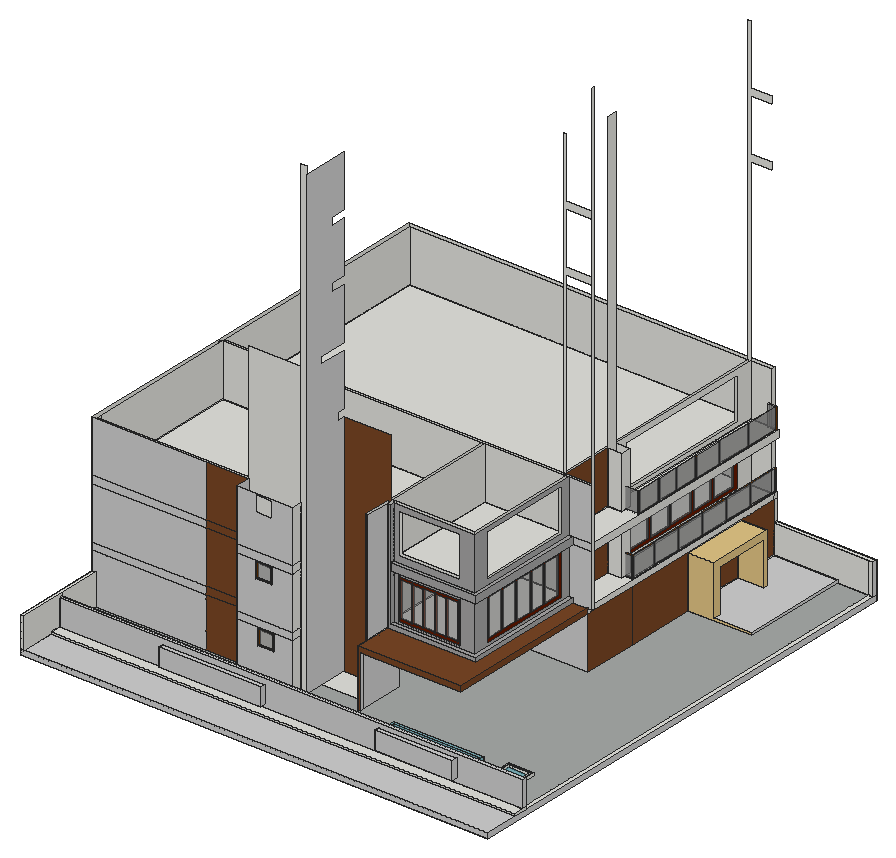
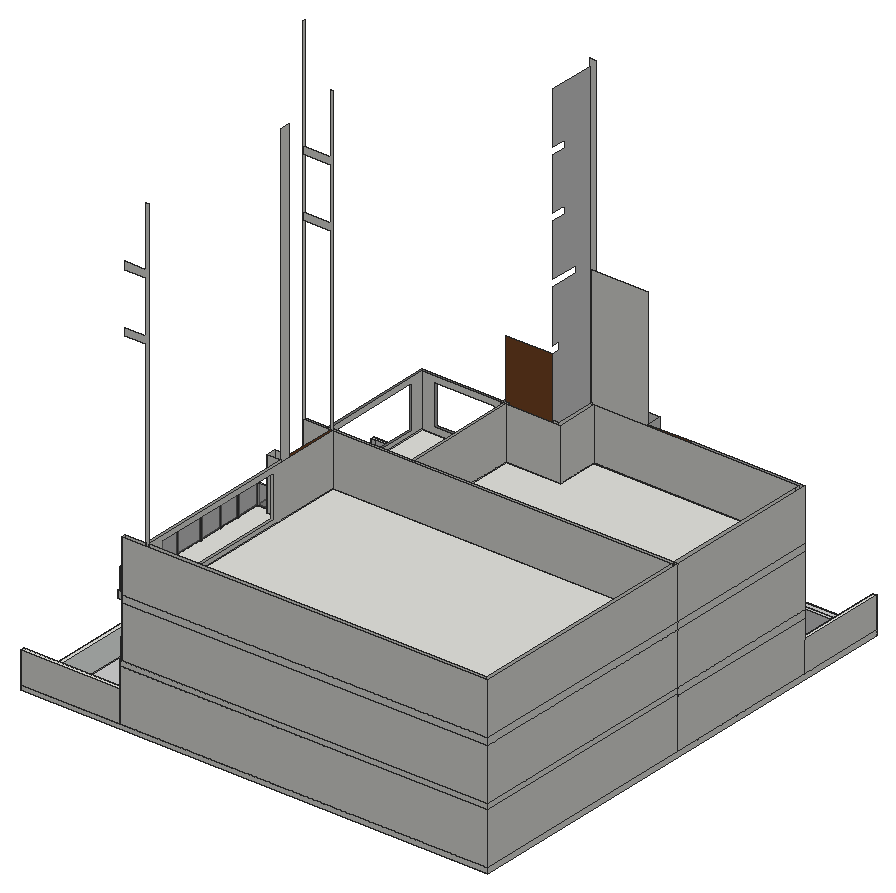
# SketchUp Ruby script. Lengths in inches.
U = 1.inch
M = Sketchup.active_model
def pt(a) = Geom::Point3d.new(a.map { |v| v * U })
def face(e, loops, mat)
  f = e.add_face(loops[0].map { |a| pt(a) })
  loops[1..].each { |l| e.add_face(l.map { |a| pt(a) }).erase! }
  f.material = f.back_material = mat if mat
  f
end
# faces: each face lists its corners as indices into pts; further lists are holes
def faces(e, pts, list, mat = nil) = list.each { |f| face(e, (f[0].is_a?(Array) ? f : [f]).map { |l| l.map { |i| pts[i] } }, mat) }
# xy, xz, yz: faces in a plane at the given z, y or x. An outline is a flat list of corners, or four numbers for a rectangle; further outlines are holes
def ring(l) = l.size == 4 ? [[l[0], l[1]], [l[2], l[1]], [l[2], l[3]], [l[0], l[3]]] : l.each_slice(2).to_a
def flat(e, list, mat, &to3) = list.each { |f| face(e, (f[0].is_a?(Array) ? f : [f]).map { |l| ring(l).map { |u, v| to3.(u, v) } }, mat) }
def xy(e, z, list, mat = nil) = flat(e, list, mat) { |x, y| [x, y, z] }
def xz(e, y, list, mat = nil) = flat(e, list, mat) { |x, z| [x, y, z] }
def yz(e, x, list, mat = nil) = flat(e, list, mat) { |y, z| [x, y, z] }
def lines(e, pts, list) = list.each { |a, b| e.add_line(pt(pts[a]), pt(pts[b])) }
# prism: a flat outline (further loops are holes) pulled along v
def prism(e, loops, v, mat = nil)
  f = face(e, loops, mat); d = Geom::Vector3d.new(v.map { |x| x * U })
  f.pushpull(f.normal.samedirection?(d) ? d.length : -d.length)
end
def box(e, o, s, mat = nil) = prism(e, [[o, [o[0] + s[0], o[1], o[2]], [o[0] + s[0], o[1] + s[1], o[2]], [o[0], o[1] + s[1], o[2]]]], [0, 0, s[2]], mat)
def at(x, y, z, deg = 0) = Geom::Transformation.translation(pt([x, y, z])) * Geom::Transformation.rotation(ORIGIN, Z_AXIS, deg.degrees)
def axes(o, x, y, z) = Geom::Transformation.new([*x, 0, *y, 0, *z, 0, *pt(o).to_a, 1])
def part(name) = M.definitions.add(name)
# library, detail: a bought-in or finely detailed component or shape, given as its bounding box
def library(name, o, s) = part(name).tap { |d| box(d.entities, o, s) }
def detail(e, o, s) = box(e.add_group.entities, o, s)
def put(e, d, t, mat = nil) = e.add_instance(d, t).tap { |i| i.material = mat if mat }
def group(e, t, mat = nil) = e.add_group.tap { |g| g.transformation = t; g.material = mat if mat }.entities
root = M.entities
M.materials.add("[Carrera Marble]").color = [207, 207, 207]
M.materials.add("[Color B08]").color = [102, 25, 0]
M.materials.add("[Color C08]").color = [102, 51, 0]
M.materials.add("[Concrete Form 4x8]").color = [167, 170, 168]
M.materials.add("[Stone Brushed Khaki]").color = [226, 197, 133]
M.materials.add("[Stone Vein Gray]").color = [166, 165, 165]
M.materials.add("[Translucent Glass Gray]").color = [128, 128, 128]
M.materials["[Translucent Glass Gray]"].alpha = 0.5
M.materials.add("[Water Pool Light]").color = [64, 149, 167]
M.materials["[Water Pool Light]"].alpha = 0.6
M.materials.add("[Wood Veneer 01]").color = [120, 70, 37]
c1 = part("Group\#1")
xy(c1.entities,0,[[0,0,21.625,260.4375]],"[Color C08]")
xy(c1.entities,20.42,[[0,20.42,21.625,240.02]],"[Color C08]")
xy(c1.entities,312.95,[[0,20.42,21.625,240.02]],"[Color C08]")
xy(c1.entities,333.375,[[0,0,21.625,260.4375]],"[Color C08]")
xz(c1.entities,0,[[0,0,21.625,333.375]],"[Color C08]")
xz(c1.entities,20.42,[[0,20.42,21.625,312.95]],"[Color C08]")
xz(c1.entities,240.02,[[0,20.42,21.625,312.95]],"[Color C08]")
xz(c1.entities,260.4375,[[0,0,21.625,333.375]],"[Color C08]")
yz(c1.entities,0,[[[0,0,260.4375,333.375],[20.42,20.42,240.02,312.95]]],"[Color C08]")
yz(c1.entities,21.625,[[[0,0,260.4375,333.375],[20.42,20.42,240.02,312.95]]],"[Color C08]")
yz(c1.entities,21.625,[[20.42,20.42,240.02,312.95]],"[Translucent Glass Gray]")
c2 = part("Group\#3")
xy(c2.entities,0,[[0,0,23.0625,440.625]],"[Color B08]")
xy(c2.entities,14.28,[[0,14.28,23.0625,92.65],[0,98.4,23.0625,173.71],[0,179.46,23.0625,261.65],[0,267.4,23.0625,340.59],[0,346.34,23.0625,426.35]],"[Color B08]")
xy(c2.entities,204.03,[[0,14.28,23.0625,92.65],[0,98.4,23.0625,173.71],[0,179.46,23.0625,261.65],[0,267.4,23.0625,340.59],[0,346.34,23.0625,426.35]],"[Color B08]")
xy(c2.entities,218.3125,[[0,0,23.0625,440.625]],"[Color B08]")
xz(c2.entities,0,[[0,0,23.0625,218.3125]],"[Color B08]")
xz(c2.entities,14.28,[[0,14.28,23.0625,204.03]],"[Color B08]")
xz(c2.entities,92.65,[[0,14.28,23.0625,204.03]],"[Color B08]")
xz(c2.entities,98.4,[[0,14.28,23.0625,204.03]],"[Color B08]")
xz(c2.entities,173.71,[[0,14.28,23.0625,204.03]],"[Color B08]")
xz(c2.entities,179.46,[[0,14.28,23.0625,204.03]],"[Color B08]")
xz(c2.entities,261.65,[[0,14.28,23.0625,204.03]],"[Color B08]")
xz(c2.entities,267.4,[[0,14.28,23.0625,204.03]],"[Color B08]")
xz(c2.entities,340.59,[[0,14.28,23.0625,204.03]],"[Color B08]")
xz(c2.entities,346.34,[[0,14.28,23.0625,204.03]],"[Color B08]")
xz(c2.entities,426.35,[[0,14.28,23.0625,204.03]],"[Color B08]")
xz(c2.entities,440.625,[[0,0,23.0625,218.3125]],"[Color B08]")
yz(c2.entities,0,[[[0,0,440.625,218.3125],[179.46,14.28,261.65,204.03],[346.34,14.28,426.35,204.03],[14.28,14.28,92.65,204.03],[98.4,14.28,173.71,204.03],[267.4,14.28,340.59,204.03]]],"[Color B08]")
yz(c2.entities,23.0625,[[[0,0,440.625,218.3125],[179.46,14.28,261.65,204.03],[346.34,14.28,426.35,204.03],[14.28,14.28,92.65,204.03],[98.4,14.28,173.71,204.03],[267.4,14.28,340.59,204.03]]],"[Color B08]")
yz(c2.entities,23.0625,[[14.28,14.28,92.65,204.03],[98.4,14.28,173.71,204.03],[179.46,14.28,261.65,204.03],[267.4,14.28,340.59,204.03],[346.34,14.28,426.35,204.03]],"[Translucent Glass Gray]")
xy(root,0,[[0,0,1080,1120.6875]])
xy(root,12,[[0,0,9,207.0625],[9,77.625,1080,109.6875],[[954.49,109.6875,1012.49,215.5625],[958.9,114.1,1008.08,211.15]],[1071,109.6875,1080,1111.6875],[362.25,171.6875,491.3125,207.0625],
  [491.3125,195.6875,506.0625,231.25],[[0,207.0625,0,573,9,573,9,322.75,491.3125,322.75,491.3125,207.0625],[9,213.0625,482.6875,316.75]],[613.75,207.0625,619.75,261.625],[9,213.0625,482.6875,316.75],[491.3125,231.25,506.0625,236.75],
  [491.3125,236.75,506.0625,301.1875],[506.0625,236.75,607.75,301.1875],[607.75,236.75,613.75,236.75,613.75,316.75,599,316.75,599,301.1875,607.75,301.1875],[613.75,261.625,619.75,316.75],[491.3125,301.1875,491.3125,322.75,613.75,322.75,613.75,316.75,599,316.75,599,301.1875],
  [[0,573,851.0625,1120.6875],[9,579,845.0625,1111.6875]],[9,579,845.0625,1111.6875],[851.0625,863.43,997.2,1111.6875],[851.0625,1111.6875,1080,1120.6875]])
xy(root,12,[[9,0,1080,77.625]],"[Carrera Marble]")
xy(root,12,[[[9,109.6875,954.49,109.6875,954.49,215.5625,1012.49,215.5625,1012.49,109.6875,1071,109.6875,1071,1111.6875,997.2,1111.6875,997.2,863.43,851.0625,863.43,851.0625,573,9,573,9,322.75,613.75,322.75,613.75,316.75,619.75,316.75,619.75,207.0625,613.75,207.0625,613.75,236.75,506.0625,236.75,506.0625,195.6875,491.3125,195.6875,491.3125,171.6875,362.25,171.6875,362.25,207.0625,9,207.0625],[733.15,114.31,932.85,161.57]]],"[Concrete Form 4x8]")
xy(root,12,[[958.9,114.1,1008.08,211.15]],"[Water Pool Light]")
xy(root,12.125,[[[728.53,109.6875,937.46,166.1875],[733.15,114.31,932.85,161.57]]])
xy(root,17,[[[954.49,109.6875,1012.49,215.5625],[958.9,114.1,1008.08,211.15]]])
xy(root,17.3125,[[9,77.625,1080,101.34],[9,101.34,1080,109.6875]])
xy(root,17.3125,[[911.25,863.43,997.2,863.43,997.2,1111.6875,851.0625,1111.6875,851.0625,1016.2,911.25,1016.2,911.25,1007.16,851.0625,1007.16,851.0625,881.2,911.25,881.2]],"[Carrera Marble]")
xy(root,23.48,[[248.24,89.97,482.8,101.34]],"[Carrera Marble]")
xy(root,25.83,[[745.92,89.41,925.92,101.34]],"[Carrera Marble]")
xy(root,44.9375,[[[728.53,109.6875,937.46,166.1875],[733.15,114.31,932.85,161.57]]],"[Water Pool Light]")
xy(root,64.42,[[248.24,89.97,482.8,101.34]],"[Carrera Marble]")
xy(root,67.2,[[745.92,89.41,925.92,101.34]],"[Carrera Marble]")
xy(root,76.6875,[[9,101.34,1080,109.6875]],"[Carrera Marble]")
xy(root,84,[[0,0,9,207.0625],[851.0625,1111.6875,1080,1120.6875]])
xy(root,88.1,[[410.19,171.6875,447.63,177.25]])
xy(root,116.5,[[851.0625,881.2,911.25,1007.16]])
xy(root,125.54,[[410.19,171.6875,447.63,177.25]])
xy(root,127,[[362.25,171.6875,491.3125,171.6875,491.3125,322.75,9,322.75,9,573,0,573,0,207.0625,362.25,207.0625]])
xy(root,132,[[619.75,207.0625,619.75,316.75,613.75,316.75,613.75,573,851.0625,573,851.0625,207.0625],[9,322.75,613.75,573],[[0,573,851.0625,1120.6875],[9,579,845.0625,1111.6875]]])
xy(root,132,[[851.0625,863.43,911.25,1016.2]],"[Stone Brushed Khaki]")
xy(root,134.8125,[[9,213.0625,482.6875,316.75]])
xy(root,138,[[9,213.0625,482.6875,316.75]])
xy(root,144,[[9,213.0625,482.6875,213.0625,482.6875,308.3125,607.75,308.3125,607.75,573,9,573],[613.75,292.25,613.75,308.3125,801.71,308.3125,801.71,573,818.15,573,818.15,292.25],[613.75,308.3125,801.71,573],[[0,573,0,1120.6875,845.0625,1120.6875,845.0625,1120.46,844.6875,1120.46,844.6875,1118.91,845.0625,1118.91,845.0625,1111.6875,797.375,1111.6875,797.375,579,851.0625,579,851.0625,573],[9,579,791.375,1111.6875]],[851.0625,573,861.375,579],
  [9,579,791.375,1111.6875],[797.375,579,851.0625,579,851.0625,1120.6875,847.375,1120.6875,847.375,708.375,828.5625,708.375,828.5625,699.0625,797.375,699.0625],[797.375,699.0625,828.5625,723.02],[828.5625,708.375,845.0625,711.125],[845.0625,708.375,847.375,711.125],
  [828.5625,711.125,845.0625,711.125,845.0625,1111.6875,797.375,1111.6875,797.375,723.02,828.5625,723.02],[845.0625,711.125,847.375,771.28],[845.0625,771.28,847.375,772.83],[845.0625,772.83,847.375,840.47],[845.0625,840.47,847.375,842.02],
  [845.0625,842.02,847.375,909.66],[845.0625,909.66,847.375,911.21],[845.0625,911.21,847.375,978.84],[845.0625,978.84,847.375,980.39],[845.0625,980.39,847.375,1048.03],
  [845.0625,1048.03,847.375,1049.58],[845.0625,1049.58,847.375,1118.91],[844.6875,1118.91,845.0625,1120.46],[845.0625,1118.91,847.375,1120.46],[845.0625,1120.46,847.375,1120.6875]])
xy(root,144,[[613.75,207.0625,851.0625,207.0625,851.0625,573,818.15,573,818.15,292.25,613.75,292.25]],"[Wood Veneer 01]")
xy(root,153.75,[[791.375,750.16,797.375,1072.78]])
xy(root,154.1875,[[621.0625,301.1875,621.0625,308.3125,801.71,308.3125,801.71,573,807.71,573,807.71,301.1875],[613.75,308.3125,801.71,573]])
xy(root,154.1875,[[621.0625,292.25,818.15,292.25,818.15,573,807.71,573,807.71,301.1875,621.0625,301.1875]],"[Stone Vein Gray]")
xy(root,158.64,[[801.71,337.86,807.71,553.05]])
xy(root,159.65,[[633.62,301.1875,774.31,308.3125]])
xy(root,192,[[844.6875,1118.91,845.0625,1120.46],[845.0625,1120.46,847.375,1120.6875]])
xy(root,192,[[828.5625,708.375,845.0625,711.125],[845.0625,708.375,847.375,711.125],[845.0625,711.125,847.375,771.28],[845.0625,771.28,847.375,772.83],[845.0625,772.83,847.375,840.47],
  [845.0625,840.47,847.375,842.02],[845.0625,842.02,847.375,909.66],[845.0625,909.66,847.375,911.21],[845.0625,911.21,847.375,978.84],[845.0625,978.84,847.375,980.39],
  [845.0625,980.39,847.375,1048.03],[845.0625,1048.03,847.375,1049.58],[845.0625,1049.58,847.375,1118.91],[845.0625,1118.91,847.375,1120.46]],"[Color C08]")
xy(root,225.25,[[406.64,171.6875,444.08,176.8125]])
xy(root,252.62,[[791.375,750.16,797.375,1072.78]])
xy(root,253.65,[[633.62,301.1875,774.31,308.3125]])
xy(root,257.64,[[801.71,337.86,807.71,553.05]])
xy(root,262.6875,[[406.64,171.6875,444.08,176.8125]])
xy(root,264,[[621.0625,301.1875,621.0625,308.3125,801.71,308.3125,801.71,573,807.71,573,807.71,301.1875],[797.375,579,797.375,699.0625,828.5625,699.0625,828.5625,723.02,797.375,723.02,797.375,1111.6875,861.375,1111.6875,861.375,579]])
xy(root,264,[[621.0625,291.875,817.65,301.1875],[807.71,301.1875,817.65,573]],"[Stone Vein Gray]")
xy(root,273,[[9,213.0625,9,573,607.75,573,607.75,308.3125,482.6875,308.3125,482.6875,213.0625]])
xy(root,275,[[613.75,308.3125,801.71,573],[9,579,791.375,1111.6875]])
xy(root,281,[[9,213.0625,482.6875,213.0625,482.6875,308.3125,607.75,308.3125,607.75,573,9,573],[621.0625,301.1875,621.0625,308.3125,801.71,308.3125,801.71,573,807.71,573,807.71,301.1875],[607.75,308.3125,613.75,573],[613.75,308.3125,801.71,573],[9,579,791.375,1111.6875],
  [797.375,579,861.375,579,861.375,1111.6875,797.375,1111.6875,797.375,723.02,828.5625,723.02,828.5625,712.3125,857.5,712.3125,857.5,1107.625,841.07,1107.625,841.07,1109.875,859.5,1109.875,859.5,710.125,828.5625,710.125,828.5625,699.0625,797.375,699.0625],[828.5625,710.125,857.5,712.3125],[857.5,710.125,859.5,712.3125],[857.5,712.3125,859.5,769],[857.5,769,859.5,770.69],
  [857.5,770.69,859.5,819.125],[857.5,819.125,859.5,820.81],[857.5,820.81,859.5,876.0625],[857.5,876.0625,859.5,877.75],[857.5,877.75,859.5,943.6875],
  [857.5,943.6875,859.5,945.38],[857.5,945.38,859.5,1026.875],[857.5,1026.875,859.5,1028.56],[857.5,1028.56,859.5,1107.625],[841.07,1107.625,857.5,1109.875],
  [857.5,1107.625,859.5,1109.875]])
xy(root,281,[[621.0625,291.875,817.65,291.875,817.65,573,807.71,573,807.71,301.1875,621.0625,301.1875]],"[Stone Vein Gray]")
xz(root,0,[[0,12,9,84]])
xz(root,0,[[0,0,1080,12]],"[Carrera Marble]")
xz(root,77.625,[[9,12,1080,17.3125]])
xz(root,89.41,[[745.92,25.83,925.92,67.2]],"[Carrera Marble]")
xz(root,89.97,[[248.24,23.48,482.8,64.42]],"[Carrera Marble]")
xz(root,101.34,[[[9,17.3125,1080,76.6875],[248.24,23.48,482.8,64.42],[745.92,25.83,925.92,67.2]]],"[Carrera Marble]")
xz(root,109.6875,[[9,12,9,17.3125,728.53,17.3125,728.53,12.125,937.46,12.125,937.46,17.3125,1071,17.3125,1071,12,1012.49,12,1012.49,17,954.49,17,954.49,12],[954.49,12,1012.49,17],[1071,12,1080,17.3125],[728.53,12.125,937.46,17.3125],[728.53,17.3125,937.46,44.9375]])
xz(root,109.6875,[[9,17.3125,9,76.6875,1071,76.6875,1071,17.3125,937.46,17.3125,937.46,44.9375,728.53,44.9375,728.53,17.3125],[1071,17.3125,1080,76.6875]],"[Carrera Marble]")
xz(root,114.1,[[958.9,12,1008.08,17]])
xz(root,114.31,[[733.15,12,932.85,12.125],[733.15,12.125,932.85,44.9375]],"[Water Pool Light]")
xz(root,161.57,[[733.15,12,932.85,12.125],[733.15,12.125,932.85,44.9375]],"[Water Pool Light]")
xz(root,166.1875,[[728.53,12.125,937.46,44.9375]])
xz(root,171.6875,[[[362.25,12,491.3125,127],[410.19,88.1,447.63,125.54]],[362.25,127,491.3125,144],[[362.25,144,491.3125,264],[406.64,225.25,444.08,262.6875]],[362.25,264,491.3125,281],[[362.25,281,491.3125,401],[406.64,362.75,444.08,400.1875]]],"[Carrera Marble]")
xz(root,176.8125,[[406.64,225.25,444.08,262.6875]])
xz(root,177.25,[[410.19,88.1,447.63,125.54]])
xz(root,195.6875,[[491.3125,12,506.0625,1103]])
xz(root,207.0625,[[0,12,9,84],[362.25,12,491.3125,675.75]])
xz(root,207.0625,[[9,12,263.74,12,263.74,127,0,127,0,84,9,84],[0,127,263.74,144],[0,144,263.74,264],[0,264,263.74,281],[0,281,263.74,401]],"[Carrera Marble]")
xz(root,207.0625,[[263.74,12,362.25,127],[613.75,12,619.75,12,619.75,132,851.0625,132,851.0625,144,613.75,144],[263.74,127,362.25,144],[263.74,144,362.25,264],[263.74,264,362.25,281],
  [263.74,281,362.25,401]],"[Wood Veneer 01]")
xz(root,211.15,[[958.9,12,1008.08,17]])
xz(root,213.0625,[[9,12,482.6875,127],[9,127,482.6875,134.8125],[9,134.8125,482.6875,138],[9,138,482.6875,144],[9,144,482.6875,264],
  [9,264,482.6875,273],[9,273,482.6875,281],[9,281,482.6875,401]])
xz(root,215.5625,[[954.49,12,1012.49,17]])
xz(root,236.75,[[607.75,12,613.75,401]])
xz(root,291.875,[[621.0625,264,817.65,281]],"[Stone Vein Gray]")
xz(root,292.25,[[613.75,144,818.15,144,818.15,154.1875,621.0625,154.1875,621.0625,401,613.75,401]],"[Stone Vein Gray]")
xz(root,301.1875,[[491.3125,12,506.0625,127],[491.3125,127,506.0625,144],[491.3125,144,506.0625,264],[491.3125,264,506.0625,281],[491.3125,281,506.0625,401]])
xz(root,301.1875,[[[621.0625,154.1875,807.71,264],[633.62,159.65,774.31,253.65]],[[621.0625,281,807.71,401],[633.62,295.58,774.31,389.58]]],"[Stone Vein Gray]")
xz(root,301.1875,[[506.0625,12,607.75,12,607.75,401,613.75,401,613.75,538,506.0625,538]],"[Wood Veneer 01]")
xz(root,308.3125,[[482.6875,144,607.75,273],[613.75,144,801.71,154.1875],[613.75,154.1875,621.0625,264],[[621.0625,154.1875,801.71,264],[633.62,159.65,774.31,253.65]],[613.75,264,621.0625,275],
  [621.0625,264,801.71,275],[482.6875,273,607.75,281],[613.75,275,621.0625,281],[621.0625,275,801.71,281],[482.6875,281,607.75,401],
  [607.75,281,613.75,401],[613.75,281,621.0625,401],[[621.0625,281,801.71,401],[633.62,295.58,774.31,389.58]]])
xz(root,316.75,[[9,12,482.6875,127],[599,12,613.75,127],[613.75,12,619.75,132],[9,127,482.6875,134.8125],[9,134.8125,482.6875,138]])
xz(root,322.75,[[9,127,491.3125,132]])
xz(root,322.75,[[9,12,491.3125,127],[491.3125,12,613.75,132]],"[Carrera Marble]")
xz(root,337.86,[[801.71,158.64,807.71,257.64]])
xz(root,553.05,[[801.71,158.64,807.71,257.64]])
xz(root,573,[[0,12,9,127],[0,127,9,132],[0,132,9,144],[9,132,613.75,144],[613.75,132,851.0625,144],
  [0,144,9,264],[9,144,607.75,264],[607.75,144,613.75,264],[613.75,144,801.71,154.1875],[801.71,144,818.15,154.1875],
  [613.75,154.1875,801.71,264],[801.71,154.1875,807.71,264],[0,264,9,281],[9,264,607.75,273],[607.75,264,613.75,281],
  [613.75,264,801.71,275],[801.71,264,817.65,281],[9,273,607.75,281],[613.75,275,801.71,281],[0,281,9,401],
  [9,281,607.75,401],[607.75,281,613.75,401],[613.75,281,801.71,401],[801.71,281,807.71,401]])
xz(root,573,[[9,12,851.0625,132],[818.15,144,861.375,144,861.375,264,807.71,264,807.71,154.1875,818.15,154.1875],[817.65,264,861.375,281],[807.71,281,861.375,401]],"[Carrera Marble]")
xz(root,579,[[9,12,845.0625,132],[9,132,9,144,791.375,144,791.375,1103,797.375,1103,797.375,966,861.375,966,861.375,949,797.375,949,797.375,829,861.375,829,861.375,812,797.375,812,797.375,144,845.0625,144,845.0625,132],[9,144,791.375,264],[797.375,144,861.375,264],[9,264,791.375,275],
  [797.375,264,861.375,281],[9,275,791.375,281],[9,281,791.375,401],[797.375,281,861.375,401]])
xz(root,699.0625,[[797.375,144,828.5625,264],[797.375,264,828.5625,281],[797.375,281,828.5625,401]])
xz(root,708.375,[[845.0625,144,847.375,192]],"[Color C08]")
xz(root,708.375,[[828.5625,144,845.0625,192]],"[Translucent Glass Gray]")
xz(root,710.125,[[857.5,281,859.5,329]],"[Color C08]")
xz(root,710.125,[[828.5625,281,857.5,329]],"[Translucent Glass Gray]")
xz(root,711.125,[[845.0625,144,847.375,192]])
xz(root,711.125,[[828.5625,144,845.0625,192]],"[Translucent Glass Gray]")
xz(root,712.3125,[[857.5,281,859.5,329]])
xz(root,712.3125,[[828.5625,281,857.5,329]],"[Translucent Glass Gray]")
xz(root,723.02,[[797.375,144,828.5625,264],[797.375,264,828.5625,281],[797.375,281,828.5625,401]])
xz(root,750.16,[[791.375,153.75,797.375,252.62]])
xz(root,769,[[857.5,281,859.5,329]])
xz(root,770.69,[[857.5,281,859.5,329]])
xz(root,771.28,[[845.0625,144,847.375,192]])
xz(root,772.83,[[845.0625,144,847.375,192]])
xz(root,819.125,[[857.5,281,859.5,329]])
xz(root,820.81,[[857.5,281,859.5,329]])
xz(root,840.47,[[845.0625,144,847.375,192]])
xz(root,842.02,[[845.0625,144,847.375,192]])
xz(root,863.43,[[851.0625,12,997.2,12,997.2,17.3125,911.25,17.3125,911.25,132,851.0625,132]],"[Stone Brushed Khaki]")
xz(root,876.0625,[[857.5,281,859.5,329]])
xz(root,877.75,[[857.5,281,859.5,329]])
xz(root,881.2,[[851.0625,17.3125,911.25,116.5]],"[Stone Brushed Khaki]")
xz(root,909.66,[[845.0625,144,847.375,192]])
xz(root,911.21,[[845.0625,144,847.375,192]])
xz(root,943.6875,[[857.5,281,859.5,329]])
xz(root,945.38,[[857.5,281,859.5,329]])
xz(root,978.84,[[845.0625,144,847.375,192]])
xz(root,980.39,[[845.0625,144,847.375,192]])
xz(root,1007.16,[[851.0625,17.3125,911.25,116.5]],"[Stone Brushed Khaki]")
xz(root,1016.2,[[851.0625,17.3125,911.25,132]],"[Stone Brushed Khaki]")
xz(root,1026.875,[[857.5,281,859.5,329]])
xz(root,1028.56,[[857.5,281,859.5,329]])
xz(root,1048.03,[[845.0625,144,847.375,192]])
xz(root,1049.58,[[845.0625,144,847.375,192]])
xz(root,1072.78,[[791.375,153.75,797.375,252.62]])
xz(root,1107.625,[[857.5,281,859.5,329]])
xz(root,1107.625,[[841.07,281,857.5,329]],"[Translucent Glass Gray]")
xz(root,1109.875,[[857.5,281,859.5,329]],"[Color C08]")
xz(root,1109.875,[[841.07,281,857.5,329]],"[Translucent Glass Gray]")
xz(root,1111.6875,[[9,12,845.0625,132],[851.0625,12,997.2,17.3125],[997.2,12,1071,12,1071,84,851.0625,84,851.0625,17.3125,997.2,17.3125],[1071,12,1080,84],[9,132,845.0625,132,845.0625,144,797.375,144,797.375,812,845.0625,812,845.0625,829,797.375,829,797.375,949,845.0625,949,845.0625,966,797.375,966,797.375,1103,791.375,1103,791.375,144,9,144],
  [9,144,791.375,264],[797.375,144,845.0625,264],[9,264,791.375,275],[797.375,264,845.0625,281],[845.0625,264,861.375,281],
  [9,275,791.375,281],[9,281,791.375,401],[797.375,281,845.0625,401]])
xz(root,1118.91,[[844.6875,144,845.0625,192],[845.0625,144,847.375,192]])
xz(root,1120.46,[[844.6875,144,845.0625,192],[845.0625,144,847.375,192]])
xz(root,1120.6875,[[0,0,1080,12],[0,12,851.0625,132],[851.0625,12,1080,84],[0,132,851.0625,144],[0,144,845.0625,264],
  [0,264,845.0625,281],[0,281,845.0625,401]])
xz(root,1120.6875,[[845.0625,144,847.375,192]],"[Color C08]")
yz(root,0,[[0,0,1120.6875,12],[0,12,207.0625,84],[207.0625,12,573,127],[573,12,1120.6875,132],[207.0625,127,573,144],
  [573,132,1120.6875,144],[207.0625,144,573,264],[573,144,1120.6875,264],[207.0625,264,573,281],[573,264,1120.6875,281],
  [207.0625,281,573,401],[573,281,1120.6875,401]])
yz(root,9,[[0,12,77.625,12,77.625,17.3125,101.34,17.3125,101.34,76.6875,109.6875,76.6875,109.6875,84,0,84],[77.625,12,109.6875,17.3125],[109.6875,12,207.0625,84],[213.0625,12,316.75,127],[579,12,1111.6875,132],
  [101.34,17.3125,109.6875,76.6875],[213.0625,127,222,134.8125],[222,127,316.75,134.8125],[322.75,127,573,132],[322.75,132,573,144],
  [579,132,1111.6875,144],[213.0625,134.8125,222,138],[222,134.8125,316.75,138],[213.0625,138,222,144],[222,138,316.75,144],
  [213.0625,144,222,264],[222,144,573,264],[579,144,1111.6875,264],[213.0625,264,222,273],[222,264,573,273],
  [579,264,1111.6875,275],[213.0625,273,222,281],[222,273,573,281],[579,275,1111.6875,281],[213.0625,281,222,401],
  [222,281,573,401],[579,281,1111.6875,401]])
yz(root,9,[[322.75,12,573,127]],"[Carrera Marble]")
yz(root,248.24,[[89.97,23.48,101.34,64.42]],"[Carrera Marble]")
yz(root,362.25,[[171.6875,12,207.0625,127],[171.6875,127,207.0625,144],[171.6875,144,207.0625,264],[171.6875,264,207.0625,281],[171.6875,281,207.0625,401]],"[Carrera Marble]")
yz(root,406.64,[[171.6875,225.25,176.8125,262.6875]])
yz(root,410.19,[[171.6875,88.1,177.25,125.54]])
yz(root,444.08,[[171.6875,225.25,176.8125,262.6875]])
yz(root,447.63,[[171.6875,88.1,177.25,125.54]])
yz(root,482.6875,[[213.0625,12,316.75,127],[213.0625,127,316.75,134.8125],[213.0625,134.8125,316.75,138],[213.0625,144,308.3125,264],[213.0625,264,308.3125,273],
  [213.0625,273,308.3125,281],[213.0625,281,308.3125,401]])
yz(root,482.8,[[89.97,23.48,101.34,64.42]],"[Carrera Marble]")
yz(root,491.3125,[[171.6875,12,195.6875,127],[195.6875,12,207.0625,127],[207.0625,12,301.1875,127],[301.1875,12,322.75,127],[171.6875,127,195.6875,144],
  [195.6875,127,207.0625,144],[207.0625,127,301.1875,144],[171.6875,144,195.6875,264],[195.6875,144,207.0625,264],[207.0625,144,301.1875,264],
  [171.6875,264,195.6875,281],[195.6875,264,207.0625,281],[207.0625,264,301.1875,281],[171.6875,281,195.6875,401],[195.6875,281,207.0625,401],
  [207.0625,281,301.1875,401]])
yz(root,506.0625,[[195.6875,12,301.1875,12,301.1875,538,282.6875,538,282.6875,555,301.1875,555,301.1875,675.75,235.5625,675.75,235.5625,692,301.1875,692,301.1875,812,267.5625,812,267.5625,829,270.6875,829,270.6875,877,272.6875,877,272.6875,829,301.1875,829,301.1875,949,267.5625,949,267.5625,966,268.8125,966,268.8125,1014,270.8125,1014,270.8125,966,301.1875,966,301.1875,1086,195.6875,1086]],"[Carrera Marble]")
yz(root,607.75,[[236.75,12,301.1875,401],[308.3125,144,573,264],[308.3125,264,573,273],[308.3125,273,548.5,281],[548.5,273,573,281],
  [308.3125,281,573,401]])
yz(root,613.75,[[207.0625,12,236.75,144],[236.75,12,316.75,127],[316.75,12,322.75,132],[236.75,127,316.75,132],[236.75,132,322.75,144],
  [322.75,132,573,144],[292.25,144,308.3125,154.1875],[308.3125,144,322.75,154.1875],[322.75,144,573,154.1875],[292.25,154.1875,308.3125,401],
  [308.3125,154.1875,573,264],[308.3125,264,573,275],[308.3125,275,318.0625,281],[318.0625,275,573,281],[308.3125,281,573,401]])
yz(root,613.75,[[236.75,144,292.25,401]],"[Carrera Marble]")
yz(root,619.75,[[207.0625,12,213.0625,132],[213.0625,12,316.75,132]],"[Carrera Marble]")
yz(root,621.0625,[[301.1875,154.1875,308.3125,264],[292.25,264,308.3125,281],[301.1875,281,308.3125,401]])
yz(root,621.0625,[[292.25,154.1875,301.1875,264],[291.875,264,292.25,281],[292.25,281,301.1875,401]],"[Stone Vein Gray]")
yz(root,633.62,[[301.1875,159.65,308.3125,253.65]])
yz(root,728.53,[[109.6875,12.125,166.1875,44.9375]])
yz(root,733.15,[[114.31,12,161.57,12.125],[114.31,12.125,161.57,44.9375]],"[Water Pool Light]")
yz(root,745.92,[[89.41,25.83,101.34,67.2]],"[Carrera Marble]")
yz(root,774.31,[[301.1875,159.65,308.3125,253.65]])
yz(root,791.375,[[[579,144,1111.6875,264],[750.16,153.75,1072.78,252.62]],[579,264,1111.6875,275],[579,275,731.0625,281],[731.0625,275,747.4375,281],[747.4375,275,1111.6875,281],
  [[579,281,1111.6875,401],[750.16,290.68,1072.78,389.56]]])
yz(root,797.375,[[699.0625,144,723.02,1086],[[723.02,144,1111.6875,264],[750.16,153.75,1072.78,252.62]],[579,264,699.0625,281],[723.02,264,1111.6875,281],[[723.02,281,1111.6875,401],[750.16,290.68,1072.78,389.56]]])
yz(root,797.375,[[579,144,699.0625,264],[579,281,699.0625,401]],"[Wood Veneer 01]")
yz(root,801.71,[[308.3125,144,573,154.1875],[[308.3125,154.1875,573,264],[337.86,158.64,553.05,257.64]],[308.3125,264,573,275],[308.3125,275,573,281],[[308.3125,281,573,401],[337.86,291.2,553.05,390.2]]])
yz(root,807.71,[[[301.1875,154.1875,573,264],[337.86,158.64,553.05,257.64]],[[301.1875,281,573,401],[337.86,291.2,553.05,390.2]]],"[Stone Vein Gray]")
yz(root,817.65,[[291.875,264,573,281]],"[Stone Vein Gray]")
yz(root,818.15,[[292.25,144,573,154.1875]],"[Stone Vein Gray]")
yz(root,828.5625,[[699.0625,144,708.375,144,708.375,192,711.125,192,711.125,144,723.02,144,723.02,264,699.0625,264],[708.375,144,711.125,192],[699.0625,264,723.02,281],[699.0625,281,710.125,281,710.125,329,712.3125,329,712.3125,281,723.02,281,723.02,401,699.0625,401],[710.125,281,712.3125,329]])
yz(root,841.07,[[1107.625,281,1109.875,329]])
yz(root,844.6875,[[1118.91,144,1120.46,192]])
yz(root,845.0625,[[579,12,1111.6875,132],[708.375,144,711.125,192],[1111.6875,144,1118.91,192],[1118.91,144,1120.46,192],[1120.46,144,1120.6875,192],
  [1111.6875,192,1120.6875,264],[1111.6875,264,1120.6875,281],[1111.6875,281,1120.6875,401]])
yz(root,845.0625,[[771.28,144,772.83,192],[840.47,144,842.02,192],[909.66,144,911.21,192],[978.84,144,980.39,192],[1048.03,144,1049.58,192]],"[Color C08]")
yz(root,845.0625,[[711.125,144,771.28,192],[772.83,144,840.47,192],[842.02,144,909.66,192],[911.21,144,978.84,192],[980.39,144,1048.03,192],
  [1049.58,144,1111.6875,192]],"[Translucent Glass Gray]")
yz(root,847.375,[[1120.46,144,1120.6875,192]])
yz(root,847.375,[[708.375,144,711.125,192],[771.28,144,772.83,192],[840.47,144,842.02,192],[909.66,144,911.21,192],[978.84,144,980.39,192],
  [1048.03,144,1049.58,192],[1118.91,144,1120.46,192]],"[Color C08]")
yz(root,847.375,[[711.125,144,771.28,192],[772.83,144,840.47,192],[842.02,144,909.66,192],[911.21,144,978.84,192],[980.39,144,1048.03,192],
  [1049.58,144,1118.91,192]],"[Translucent Glass Gray]")
yz(root,851.0625,[[[863.43,12,1111.6875,12,1111.6875,17.3125,1016.2,17.3125,1016.2,132,863.43,132],[881.2,17.3125,1007.16,116.5]],[1111.6875,12,1120.6875,84],[1111.6875,84,1120.6875,132],[573,132,1111.6875,144],[1111.6875,132,1120.6875,144]])
yz(root,851.0625,[[573,12,702.65,132],[702.65,12,863.43,132],[881.2,17.3125,1007.16,116.5],[1016.2,17.3125,1111.6875,132],[207.0625,132,573,144]],"[Wood Veneer 01]")
yz(root,857.5,[[710.125,281,712.3125,329],[1107.625,281,1109.875,329]])
yz(root,857.5,[[769,281,770.69,329],[819.125,281,820.81,329],[876.0625,281,877.75,329],[943.6875,281,945.38,329],[1026.875,281,1028.56,329]],"[Color C08]")
yz(root,857.5,[[712.3125,281,769,329],[770.69,281,819.125,329],[820.81,281,876.0625,329],[877.75,281,943.6875,329],[945.38,281,1026.875,329],
  [1028.56,281,1107.625,329]],"[Translucent Glass Gray]")
yz(root,859.5,[[710.125,281,712.3125,329],[769,281,770.69,329],[819.125,281,820.81,329],[876.0625,281,877.75,329],[943.6875,281,945.38,329],
  [1026.875,281,1028.56,329],[1107.625,281,1109.875,329]],"[Color C08]")
yz(root,859.5,[[712.3125,281,769,329],[770.69,281,819.125,329],[820.81,281,876.0625,329],[877.75,281,943.6875,329],[945.38,281,1026.875,329],
  [1028.56,281,1107.625,329]],"[Translucent Glass Gray]")
yz(root,861.375,[[573,144,579,1223],[579,264,1111.6875,281]])
yz(root,911.25,[[863.43,17.3125,881.2,17.3125,881.2,116.5,1007.16,116.5,1007.16,17.3125,1016.2,17.3125,1016.2,132,863.43,132]],"[Stone Brushed Khaki]")
yz(root,925.92,[[89.41,25.83,101.34,67.2]],"[Carrera Marble]")
yz(root,932.85,[[114.31,12.125,161.57,44.9375]])
yz(root,932.85,[[114.31,12,161.57,12.125]],"[Water Pool Light]")
yz(root,937.46,[[109.6875,12.125,166.1875,44.9375]],"[Water Pool Light]")
yz(root,954.49,[[109.6875,12,215.5625,17]])
yz(root,958.9,[[114.1,12,211.15,17]])
yz(root,997.2,[[863.43,12,1111.6875,17.3125]],"[Carrera Marble]")
yz(root,1008.08,[[114.1,12,211.15,17]])
yz(root,1012.49,[[109.6875,12,215.5625,17]])
yz(root,1080,[[77.625,12,109.6875,17.3125]])
yz(root,1080,[[0,0,1120.6875,12],[1111.6875,12,1120.6875,84],[101.34,17.3125,109.6875,76.6875]],"[Carrera Marble]")
p = [[619.75,261.625,132],[619.75,261.625,144],[845.0625,595.6875,132],[845.0625,595.6875,144],[613.75,261.625,132],[482.6875,316.75,144],
  [482.6875,316.75,138],[491.3125,322.75,132],[491.3125,322.75,144],[599,316.75,127],[599,301.1875,127],[851.0625,702.65,12],
  [851.0625,702.65,3.25]]
lines(root,p,[[0,1],[2,3],[4,0],[5,6],[7,8],[9,10],[11,12]])
put(root,c1,axes([410.19,171.6875,88.1],[0,0.11448,0],[0.14375,0,0],[0,0,0.1123]))
put(root,c2,axes([792.53,750.55,153.75],[0.21,0,0],[0,0.7313,0],[0,0,0.45291]))
put(root,c2,axes([802.87,337.86,158.64],[0.126,0,0],[0,0.48837,0],[0,0,0.45348]))
put(root,c2,axes([633.62,303.92,159.65],[0,-0.11844,0],[0.31929,0,0],[0,0,0.43058]))
put(root,c1,axes([406.64,171.6875,225.25],[0,0.11448,0],[0.14375,0,0],[0,0,0.1123]))
